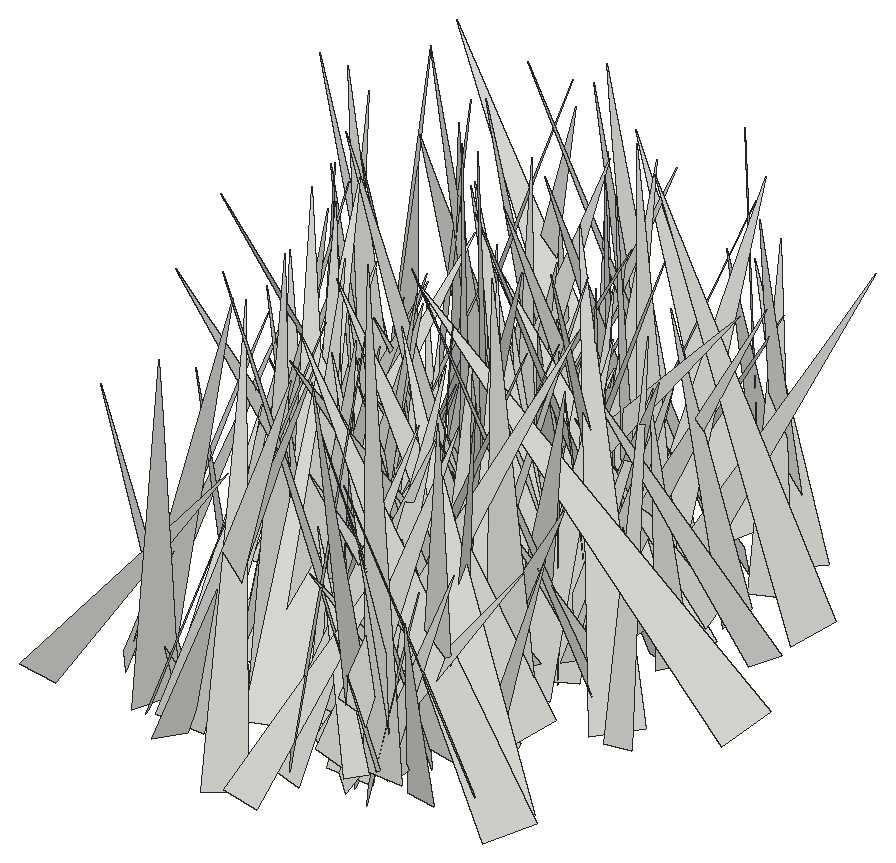
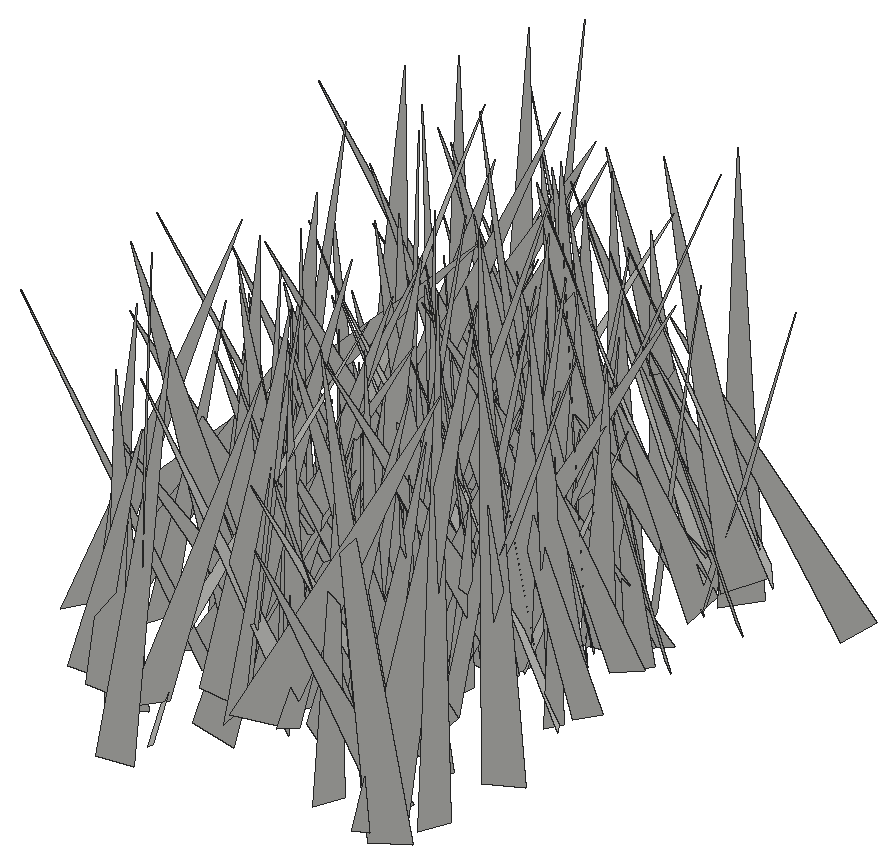
# SketchUp Ruby script. Lengths in inches.
U = 1.inch
M = Sketchup.active_model
def pt(a) = Geom::Point3d.new(a.map { |v| v * U })
def face(e, loops, mat)
  f = e.add_face(loops[0].map { |a| pt(a) })
  loops[1..].each { |l| e.add_face(l.map { |a| pt(a) }).erase! }
  f.material = f.back_material = mat if mat
  f
end
# faces: each face lists its corners as indices into pts; further lists are holes
def faces(e, pts, list, mat = nil) = list.each { |f| face(e, (f[0].is_a?(Array) ? f : [f]).map { |l| l.map { |i| pts[i] } }, mat) }
# xy, xz, yz: faces in a plane at the given z, y or x. An outline is a flat list of corners, or four numbers for a rectangle; further outlines are holes
def ring(l) = l.size == 4 ? [[l[0], l[1]], [l[2], l[1]], [l[2], l[3]], [l[0], l[3]]] : l.each_slice(2).to_a
def flat(e, list, mat, &to3) = list.each { |f| face(e, (f[0].is_a?(Array) ? f : [f]).map { |l| ring(l).map { |u, v| to3.(u, v) } }, mat) }
def xy(e, z, list, mat = nil) = flat(e, list, mat) { |x, y| [x, y, z] }
def xz(e, y, list, mat = nil) = flat(e, list, mat) { |x, z| [x, y, z] }
def yz(e, x, list, mat = nil) = flat(e, list, mat) { |y, z| [x, y, z] }
def lines(e, pts, list) = list.each { |a, b| e.add_line(pt(pts[a]), pt(pts[b])) }
# prism: a flat outline (further loops are holes) pulled along v
def prism(e, loops, v, mat = nil)
  f = face(e, loops, mat); d = Geom::Vector3d.new(v.map { |x| x * U })
  f.pushpull(f.normal.samedirection?(d) ? d.length : -d.length)
end
def box(e, o, s, mat = nil) = prism(e, [[o, [o[0] + s[0], o[1], o[2]], [o[0] + s[0], o[1] + s[1], o[2]], [o[0], o[1] + s[1], o[2]]]], [0, 0, s[2]], mat)
def at(x, y, z, deg = 0) = Geom::Transformation.translation(pt([x, y, z])) * Geom::Transformation.rotation(ORIGIN, Z_AXIS, deg.degrees)
def axes(o, x, y, z) = Geom::Transformation.new([*x, 0, *y, 0, *z, 0, *pt(o).to_a, 1])
def part(name) = M.definitions.add(name)
# library, detail: a bought-in or finely detailed component or shape, given as its bounding box
def library(name, o, s) = part(name).tap { |d| box(d.entities, o, s) }
def detail(e, o, s) = box(e.add_group.entities, o, s)
def put(e, d, t, mat = nil) = e.add_instance(d, t).tap { |i| i.material = mat if mat }
def group(e, t, mat = nil) = e.add_group.tap { |g| g.transformation = t; g.material = mat if mat }.entities
root = M.entities
c1 = part("fur_instance\#9")
p = [[0.8125,0,1.79],[0.67,-0.02,1.48],[0,-0.11,0],[0,0.11,0]]
faces(c1.entities,p,[[0,1,2,3]])
put(root,c1,axes([78.76,74.87,-28.22],[-4.90354,-1.85753,0.89414],[-1.8937,4.97041,-0.05944],[0.81474,0.37312,5.24324]))
put(root,c1,axes([74.27,73.58,-28.22],[3.74419,-3.98525,0.35569],[-3.51637,-3.04515,2.89653],[1.90889,2.20738,4.63803]))
put(root,c1,axes([81.04,83.26,-27.1],[-7.866,-1.33504,0.19154],[-1.32695,7.45779,-2.51268],[-0.24134,2.50839,7.5725]))
put(root,c1,axes([76.8125,81.12,-27.1],[-1.32926,4.80497,0.97182],[4.66035,1.55098,-1.29408],[1.52094,-0.553,4.81456]))
put(root,c1,axes([78.3,80.58,-27.1],[-1.55203,4.86816,1.43833],[5.0761,1.479,0.47157],[-0.03172,-1.51332,5.08777]))
put(root,c1,axes([78.59,81.8,-27.1],[-7.01527,0.64484,2.20419],[0.06996,7.14138,-1.86657],[2.29551,1.75305,6.79307]))
put(root,c1,axes([78.87,84.04,-27.1],[-4.6642,0.46344,0.8289],[0.1067,4.38406,-1.85075],[0.94364,1.79496,4.30631]))
put(root,c1,axes([75.77,77.2,-27.1],[4.35224,4.23695,0.82253],[4.28263,-4.09432,-1.57033],[0.53605,-1.68972,5.86752]))
put(root,c1,axes([76.0625,80.16,-27.1],[4.67492,4.49227,1.13099],[4.6277,-4.45606,-1.42912],[0.20972,-1.8104,6.324]))
put(root,c1,axes([76.66,90.22,-28.22],[7.73874,0.04549,1.82687],[0.5794,-7.60007,-2.26513],[-1.73315,-2.33761,7.39995]))
put(root,c1,axes([77.17,89.34,-27.1],[4.35751,-1.25814,0.68683],[-1.21703,-4.4086,-0.35441],[-0.75729,-0.15444,4.52164]))
put(root,c1,axes([77.69,91.51,-28.22],[6.63906,-4.24471,1.17982],[-3.75911,-6.57064,-2.48644],[-2.29753,-1.51516,7.47745]))
put(root,c1,axes([79.32,82.79,-27.1],[-2.85386,-2.94003,0.13695],[-2.93623,2.85714,0.14971],[0.2028,-0.00613,4.09462]))
put(root,c1,axes([78.6,75.36,-28.22],[-5.00496,1.9066,1.35129],[1.19771,4.83542,-2.3864],[2.00664,1.8693,4.79477]))
put(root,c1,axes([79.34,83.54,-27.1],[-7.46216,1.5868,2.36089],[1.65538,7.81249,-0.01867],[2.31332,-0.47194,7.62898]))
put(root,c1,axes([77.67,83.45,-28.22],[3.91592,-0.46866,0.80636],[-0.26131,-3.89224,-0.99321],[-0.89531,-0.91384,3.81675]))
put(root,c1,axes([77.03,74.16,-27.1],[4.58247,4.01128,0.43645],[4.00699,-4.60163,0.22113],[-0.47421,-0.12046,6.08609]))
put(root,c1,axes([79.05,75.29,-27.1],[-4.90566,2.32822,0.51514],[1.6552,4.17303,-3.098],[1.71648,2.62995,4.45965]))
put(root,c1,axes([77.82,79.22,-28.22],[3.13443,-2.25979,0.73802],[-2.32723,-3.16608,0.18952],[-0.4851,0.5876,3.85946]))
put(root,c1,axes([81.81,83.98,-28.22],[-3.80092,-6.72254,0.0507],[-6.48684,3.65215,-2.05545],[-1.76524,1.05421,7.4441]))
put(root,c1,axes([76,83.94,-27.1],[0.54416,-5.67013,1.84078],[-5.27926,0.40028,2.79359],[2.76917,1.87733,4.9641]))
put(root,c1,axes([78.63,80.76,-27.1],[-4.89725,-3.9807,3.26033],[-4.56553,5.43754,-0.21877],[2.37312,2.24631,6.30723]))
put(root,c1,axes([76.62,87.05,-28.22],[-0.13317,-8.12567,1.45261],[-7.87911,0.55826,2.40046],[2.46092,1.34765,7.76415]))
put(root,c1,axes([77.31,75.09,-27.1],[6.16664,-2.56617,1.31423],[-2.70082,-6.22755,0.51287],[-1.00896,0.98602,6.65955]))
put(root,c1,axes([79.95,81.62,-27.1],[4.59054,6.55576,1.84003],[6.00661,-4.94402,2.62946],[-3.20693,0.124,7.5589]))
put(root,c1,axes([79.47,85.91,-27.1],[-3.91198,-5.41617,1.52932],[-5.50053,4.07361,0.35664],[1.19076,1.02376,6.67167]))
put(root,c1,axes([78.52,80.5625,-27.1],[2.84043,2.51238,0.82611],[2.52394,-2.93724,0.2547],[-0.79009,-0.35083,3.78354]))
put(root,c1,axes([79.33,76.82,-28.22],[-4.6895,-2.45579,1.69505],[-2.43913,4.97359,0.45768],[1.71894,0.35769,5.27378]))
put(root,c1,axes([77.96,74.4,-28.22],[6.0824,-3.06076,1.36011],[-2.97573,-6.23245,-0.71791],[-1.53726,-0.04598,6.77115]))
put(root,c1,axes([78.59,80.53,-27.1],[4.23217,0.79223,1.75299],[1.35483,-4.23497,-1.35698],[-1.36567,-1.74623,4.08626]))
put(root,c1,axes([77.05,91.76,-28.22],[0.9927,-7.18833,2.00129],[-7.23058,-0.4281,2.04891],[1.84279,2.19257,6.96128]))
put(root,c1,axes([78.36,78.8,-28.22],[7.07212,-1.1156,2.41076],[-1.38462,-7.39913,0.63784],[-2.26697,1.03896,7.1311]))
put(root,c1,axes([80.45,81.93,-27.1],[-6.61174,-0.50833,1.66504],[-0.62205,6.79727,-0.39495],[1.62598,0.53342,6.61948]))
put(root,c1,axes([80.125,88.79,-27.1],[-0.83956,4.61048,2.28414],[5.1209,0.52371,0.82514],[-0.50027,-2.37653,4.61309]))
put(root,c1,axes([79.41,74.06,-27.1],[-0.73079,4.32054,0.1844],[4.30671,0.74406,-0.36572],[0.39156,-0.12013,4.36662]))
put(root,c1,axes([79.86,87.125,-28.22],[0.81104,4.54834,1.26147],[4.65262,-0.98593,0.56355],[-0.7949,-1.13006,4.58559]))
put(root,c1,axes([77.7,82.79,-27.1],[3.43659,4.37627,1.35344],[4.55407,-3.08156,-1.59944],[0.49399,-2.03617,5.32951]))
put(root,c1,axes([80.07,85.16,-28.22],[-4.55771,-1.35516,1.4154],[-1.26006,4.77117,0.51063],[1.50069,-0.10962,4.72742]))
put(root,c1,axes([79.25,74.73,-28.22],[5.51307,6.12337,0.96272],[5.81555,-5.55551,2.03274],[-2.14519,0.67601,7.98483]))
put(root,c1,axes([78.45,90.6,-28.22],[1.64053,-3.56149,0.70323],[-3.59089,-1.47867,0.88831],[0.53314,0.99969,3.81922]))
put(root,c1,axes([80.87,81.26,-27.1],[-6.78403,-3.28205,0.63683],[-2.89291,6.48484,2.60352],[1.67585,-2.09175,7.07224]))
put(root,c1,axes([83.32,90.05,-27.1],[-5.71693,5.39586,0.3581],[5.20349,5.34707,2.50186],[-1.47216,-2.05434,7.45247]))
put(root,c1,axes([80.95,83.7,-28.22],[-4.35702,1.54483,0.37411],[1.45493,4.3157,-0.87633],[0.64002,0.7059,4.53896]))
put(root,c1,axes([77.67,83.2,-28.22],[4.98455,3.49636,0.32674],[3.50629,-4.92427,-0.79656],[0.19289,-0.83908,6.03621]))
put(root,c1,axes([79.35,72.3,-27.1],[3.38601,2.0667,0.33408],[1.88033,-3.28152,1.24252],[-0.92044,0.89903,3.76728]))
put(root,c1,axes([80.5,80.37,-28.22],[-3.8802,0.07929,1.10053],[0.11582,4.03064,0.11798],[1.09728,-0.14508,3.87922]))
put(root,c1,axes([79.5,82.96,-27.1],[6.78257,3.66457,1.14232],[2.83952,-6.35069,3.51329],[-2.58286,2.6414,6.86216]))
put(root,c1,axes([77.94,90.25,-28.22],[4.34648,-1.55951,0.20323],[-1.53377,-4.07129,1.56122],[0.34774,1.53551,4.34586]))
put(root,c1,axes([78.38,78.01,-28.22],[-0.73588,7.38124,0.25307],[6.98236,0.77818,-2.39362],[2.40696,-0.00075,7.02103]))
put(root,c1,axes([80.36,83.2,-28.22],[5.2038,5.70361,2.35891],[5.67233,-5.63566,1.11317],[-2.43315,-0.93989,7.64013]))
put(root,c1,axes([79.96,90.97,-28.22],[4.81176,-1.3762,1.70282],[-1.26945,-5.10354,-0.53746],[-1.78382,-0.0803,4.97575]))
put(root,c1,axes([82.38,88.38,-28.22],[-3.32037,-5.8988,2.51801],[-6.36421,2.67847,-2.11746],[-0.7956,3.19234,6.42939]))
put(root,c1,axes([78.86,89.73,-28.22],[2.1882,-4.93746,0.79161],[-4.93819,-1.99768,1.19031],[0.78701,1.19336,5.26781]))
put(root,c1,axes([81.52,86.59,-28.22],[1.26749,-5.25605,0.55346],[-5.00773,-1.37633,-1.60227],[-1.68968,0.13629,5.16385]))
put(root,c1,axes([80.47,76.65,-28.22],[-0.16128,6.84934,2.86842],[7.42417,0.20732,-0.07764],[0.15166,-2.86546,6.8508]))
put(root,c1,axes([78.57,75.2,-27.1],[5.68273,3.19615,0.64935],[3.24559,-5.67036,-0.49352],[-0.32122,-0.74969,6.50117]))
put(root,c1,axes([81.94,85.8125,-27.1],[-7.67624,-2.38765,2.18106],[-2.53698,7.93,-0.24775],[2.0054,0.89261,8.03519]))
put(root,c1,axes([81.24,81.71,-27.1],[-0.33834,3.74046,0.53618],[3.75079,0.26714,0.50319],[-0.45836,-0.57497,3.72187]))
put(root,c1,axes([80.7,85.74,-27.1],[3.27584,-2.78093,0.2499],[-2.38988,-2.99185,-1.96583],[-1.44378,-1.35736,3.82103]))
put(root,c1,axes([82.16,76.27,-28.22],[-5.1988,6.07272,1.14347],[6.1224,5.26442,-0.12263],[0.83765,-0.78798,7.99315]))
put(root,c1,axes([79.35,82.78,-27.1],[3.86855,-0.79855,0.19754],[-0.81455,-3.85123,0.38332],[-0.11496,0.41562,3.93147]))
put(root,c1,axes([81.46,82.02,-28.22],[-0.43977,4.5707,0.64422],[4.59918,0.3789,0.45132],[-0.39225,-0.6818,4.56957]))
put(root,c1,axes([79.14,88.125,-27.1],[2.35297,-5.60644,2.50548],[-6.03434,-1.6135,2.05656],[1.13856,3.03489,5.72182]))
put(root,c1,axes([82.9,76,-27.1],[-6.0397,-1.24718,1.08354],[-1.47294,5.92489,-1.39057],[0.74831,1.59618,6.00831]))
put(root,c1,axes([79.6875,79.56,-27.1],[5.0608,-1.8582,0.79428],[-1.91101,-5.09708,0.2516],[-0.65714,0.51221,5.38529]))
put(root,c1,axes([79.54,73.09,-28.22],[6.41211,-0.61612,1.30158],[-0.93497,-6.2989,1.62436],[-1.09524,1.77006,6.23347]))
put(root,c1,axes([82.84,71.48,-28.22],[-6.61706,2.95045,0.41304],[2.75432,6.44194,-1.89112],[1.13554,1.56763,6.99387]))
put(root,c1,axes([79.96,87.74,-27.1],[4.40688,2.08061,0.00975],[2.02682,-4.29803,1.08102],[-0.47012,0.97349,4.75194]))
put(root,c1,axes([79.34,73.8125,-28.22],[2.98572,-5.88102,1.99527],[-6.13329,-2.44486,1.97166],[0.97482,2.63026,6.29392]))
put(root,c1,axes([83.88,82.41,-27.1],[-7.9003,-1.05971,0.99848],[-1.05239,7.96314,0.1246],[1.0062,0.00826,7.97008]))
put(root,c1,axes([79.52,80.73,-28.22],[4.01839,-5.64573,1.18023],[-5.73753,-3.76564,1.52164],[0.58986,1.83314,6.76065]))
put(root,c1,axes([82.41,85.7,-28.22],[1.55743,6.34801,1.89562],[6.44853,-1.89902,1.06134],[-1.51893,-1.55328,6.44953]))
put(root,c1,axes([82.76,73.87,-27.1],[-4.41357,6.91206,0.00056],[6.86097,4.38103,-0.99489],[0.83882,0.53496,8.14041]))
put(root,c1,axes([82.54,76.4,-28.22],[-1.87564,7.62096,1.95831],[7.8685,1.80971,0.49369],[-0.027,-2.0194,7.83284]))
put(root,c1,axes([82.36,89.85,-27.1],[-3.76395,0.54517,1.33918],[0.93594,3.7652,1.09781],[1.1021,-1.33566,3.64133]))
put(root,c1,axes([79.06,89.62,-28.22],[5.13352,5.29295,1.04527],[5.31008,-4.70157,-2.27141],[0.95446,-2.31104,7.01492]))
put(root,c1,axes([83.82,77.97,-28.22],[-1.56415,5.71782,0.81541],[5.62888,1.31989,1.54221],[-1.29382,-1.17019,5.72377]))
put(root,c1,axes([80.8125,79.18,-27.1],[3.7872,-0.0255,0.26622],[0.02172,-3.73751,-0.66706],[-0.26655,-0.66693,3.72808]))
put(root,c1,axes([82.58,75.08,-27.1],[-5.70861,3.53079,2.01517],[3.32922,6.05385,-1.17592],[2.33318,0.00055,6.60847]))
put(root,c1,axes([82.73,80.1875,-27.1],[0.53786,-3.60504,0.14249],[-3.55289,-0.5543,-0.6129],[-0.62738,0.04841,3.59304]))
put(root,c1,axes([80.73,89.14,-27.1],[5.43533,-0.93824,0.08866],[-0.80913,-4.91198,-2.3767],[-0.48317,-2.32876,4.97739]))
put(root,c1,axes([81.07,77.69,-28.22],[2.15737,-6.51602,1.69287],[-6.69271,-1.88316,1.28061],[0.7294,1.99342,6.74336]))
put(root,c1,axes([86.87,73.8125,-27.1],[-6.97142,-3.26118,0.0354],[-2.96258,6.29742,-3.28677],[-1.3637,2.99072,6.9594]))
put(root,c1,axes([81.07,85.01,-28.22],[5.44463,0.12063,0.24069],[0.04962,-5.23956,1.50366],[-0.26462,1.49964,5.23426]))
put(root,c1,axes([80.71,84.64,-27.1],[6.6655,-1.52718,0.22941],[-1.49066,-6.62814,-0.81212],[-0.40351,-0.74118,6.78982]))
put(root,c1,axes([84.09,90.09,-27.1],[-6.8866,-1.44069,2.04712],[-1.4724,7.17733,0.09795],[2.02444,0.3193,7.035]))
put(root,c1,axes([84.39,80.79,-28.22],[-7.45834,-2.27512,2.73301],[-2.96816,7.48025,-1.87304],[1.95846,2.67246,7.56933]))
put(root,c1,axes([83.48,85.23,-27.1],[-3.08367,2.72536,1.78242],[3.08151,3.23588,0.38343],[1.05304,-1.48834,4.09751]))
put(root,c1,axes([84.33,87.04,-28.22],[-6.55431,0.09701,1.7896],[-0.34688,6.588,-1.62754],[1.75834,1.66126,6.34976]))
put(root,c1,axes([83.85,84.11,-28.22],[0.37183,-3.94608,0.38846],[-3.8933,-0.43727,-0.71534],[-0.75144,0.31297,3.89847]))
put(root,c1,axes([84.875,89.6875,-27.1],[-1.73257,6.85044,2.42635],[7.20837,1.30251,1.46979],[-0.92468,-2.68187,6.91158]))
put(root,c1,axes([82.66,84.1,-28.22],[-0.63847,4.33122,0.11328],[4.14955,0.64421,-1.24344],[1.2464,0.07394,4.19773]))
put(root,c1,axes([83.06,80.74,-27.1],[4.36466,2.86173,1.95624],[3.18404,-4.55325,-0.44325],[-1.3705,-1.46462,5.20032]))
put(root,c1,axes([85.26,83.08,-27.1],[-5.2406,4.407,1.34408],[4.57378,5.22157,0.71269],[0.55566,-1.41624,6.81011]))
put(root,c1,axes([87.54,89.21,-27.1],[-7.14593,-4.06809,0.00282],[-3.91681,6.87864,-2.22635],[-1.09909,1.93614,7.91562]))
put(root,c1,axes([84.1,84.14,-28.22],[-3.37943,-0.96857,0.84627],[-0.6019,3.29348,1.36586],[1.13667,-1.13567,3.23931]))
put(root,c1,axes([84.03,87.23,-27.1],[-0.63245,-3.70623,0.66325],[-3.76509,0.62047,-0.12308],[-0.01169,0.67448,3.75779]))
put(root,c1,axes([85.34,88.22,-28.22],[-0.04463,-6.97717,1.39975],[-6.92736,-0.27772,-1.60522],[-1.62845,1.37265,6.79015]))
put(root,c1,axes([83.9,88.21,-28.22],[3.78368,4.97369,3.03573],[5.56614,-4.15585,-0.12867],[-1.72376,-2.50217,6.24798]))
put(root,c1,axes([84.41,86.54,-28.22],[-2.40754,3.72637,1.88833],[4.14407,2.40561,0.53634],[0.52762,-1.89079,4.40391]))
put(root,c1,axes([82.66,77.62,-27.1],[-2.78435,-5.66723,3.39056],[-5.97834,3.72634,1.319],[2.80584,2.3158,6.17497]))
put(root,c1,axes([81.21,81.07,-28.22],[7.73901,0.54751,0.09462],[0.50511,-7.48314,1.98706],[-0.23147,1.9758,7.49957]))
put(root,c1,axes([85.05,89.98,-28.22],[-0.92127,-7.60318,0.93237],[-7.64439,0.85236,-0.60268],[-0.49091,0.99576,7.63504]))
put(root,c1,axes([83.86,76.51,-28.22],[-3.43259,1.11019,2.13702],[1.24058,4.00441,-0.08763],[2.06406,-0.56053,3.60659]))
put(root,c1,axes([86.41,91.24,-27.1],[-6.01632,2.22797,0.81671],[2.32649,5.97644,0.83455],[0.46722,-1.07014,6.36109]))
put(root,c1,axes([86.2,80.86,-27.1],[2.18391,-6.70079,0.42323],[-6.08063,-2.16263,-2.86325],[-2.84706,-0.52116,6.43986]))
put(root,c1,axes([86.59,88.07,-28.22],[-2.69174,-3.80387,0.07847],[-3.66679,2.56798,-1.29661],[-1.01502,0.8106,4.47591]))
put(root,c1,axes([82.83,88.76,-27.1],[5.42276,2.60915,0.23648],[2.58182,-5.41452,0.53583],[-0.44475,0.3811,5.9939]))
put(root,c1,axes([85.51,80.41,-27.1],[-6.98093,-2.98191,2.95578],[-3.56155,7.24267,-1.10492],[2.22346,2.23913,7.51028]))
put(root,c1,axes([86.6,75.18,-27.1],[-5.80582,1.67481,0.45332],[1.66732,5.82342,-0.1609],[0.48013,0.02943,6.04042]))
put(root,c1,axes([85.71,84.58,-27.1],[-3.47043,-1.20582,0.35373],[-1.16309,3.47557,0.43669],[0.47575,-0.29913,3.64791]))
put(root,c1,axes([84.6,77.88,-27.1],[2.87799,2.64757,1.74089],[2.94858,-3.09885,-0.16173],[-1.16026,-1.30792,3.90721]))
put(root,c1,axes([83.55,73.28,-28.22],[0.68062,5.93772,0.86921],[5.89172,-0.495,-1.23203],[1.14003,-0.98679,5.84823]))
put(root,c1,axes([83.43,78.71,-28.22],[5.03516,3.5658,0.22039],[3.50469,-5.00395,0.89105],[-0.69327,0.6016,6.10523]))
put(root,c1,axes([85.06,83.76,-27.1],[-1.60634,4.05647,0.77587],[4.09581,1.67158,-0.25963],[0.53033,-0.623,4.35521]))
put(root,c1,axes([83.49,71.4,-28.22],[-2.11402,4.56513,0.60738],[3.84978,2.11854,-2.52378],[2.52756,0.59144,4.35202]))
put(root,c1,axes([84.43,72.55,-27.1],[5.20843,4.28763,1.83578],[4.29945,-5.48037,0.60158],[-1.80791,-0.68076,6.71935]))
put(root,c1,axes([86.52,73,-27.1],[-0.98772,3.5916,0.11089],[3.35733,0.88143,1.35606],[-1.28071,-0.45933,3.46934]))
put(root,c1,axes([88.375,86.31,-28.22],[-6.39943,2.86094,0.01202],[2.71801,6.07041,2.2137],[-0.89308,-2.0256,6.65111]))
put(root,c1,axes([85.47,78.5,-27.1],[-4.49774,2.41965,1.22715],[2.26445,4.65664,-0.88215],[1.49428,0.22634,5.03052]))
put(root,c1,axes([82.98,75.65,-27.1],[2.29321,-4.71361,1.70331],[-4.8602,-1.63403,2.02152],[1.22385,2.34308,4.83635]))
put(root,c1,axes([84.94,86.23,-27.1],[-5.03968,3.97301,2.20808],[3.85689,5.48236,-1.06156],[2.40517,-0.46656,6.329]))
put(root,c1,axes([87.78,85.45,-28.22],[-4.08084,-6.31933,0.93728],[-6.28934,3.77891,-1.90517],[-1.12095,1.80323,7.27719]))
put(root,c1,axes([85.7,84.49,-27.1],[-3.90689,0.46662,1.17538],[0.26281,4.03296,-0.72751],[1.23701,0.61693,3.86682]))
put(root,c1,axes([85.11,86.32,-28.22],[1.4103,3.34023,0.25009],[3.32818,-1.428,0.30438],[-0.37801,-0.11091,3.61295]))
put(root,c1,axes([86.65,77.71,-27.1],[-4.86866,0.51762,1.11395],[0.97098,4.41082,2.19421],[0.75234,-2.34296,4.3769]))
put(root,c1,axes([86.41,82.62,-28.22],[-5.37291,2.30629,0.61766],[1.96946,5.14098,-2.06404],[1.34972,1.6793,5.47055]))
put(root,c1,axes([87.89,77.5,-28.22],[-5.88175,-1.50758,0.15009],[-1.51502,5.85044,-0.60606],[-0.00586,0.62434,6.04156]))
put(root,c1,axes([86.38,77.99,-28.22],[-4.21387,-1.59887,0.24339],[-1.27519,3.70248,2.24451],[0.99474,-2.02671,3.90836]))
put(root,c1,axes([85.84,84.82,-28.22],[-3.08736,-2.6391,1.38175],[-2.74426,3.29386,0.15946],[1.15895,0.7691,4.05847]))
put(root,c1,axes([83.46,77.81,-27.1],[6.47298,0.85818,0.33872],[0.84258,-6.4766,0.30739],[-0.37587,0.26066,6.52238]))
put(root,c1,axes([85.18,75.14,-28.22],[-6.68782,-2.79113,3.18251],[-2.04813,7.34131,2.13449],[3.70459,-0.98003,6.92541]))
put(root,c1,axes([86.66,78.6875,-28.22],[-3.82919,5.78151,1.38736],[5.88668,3.91838,-0.08139],[0.83523,-1.11076,6.93412]))
put(root,c1,axes([85.125,74.44,-28.22],[-1.23701,6.48468,1.94316],[6.59867,1.59608,-1.12573],[1.51147,-1.6609,6.50492]))
put(root,c1,axes([87.62,75.09,-27.1],[-4.41159,-3.54695,0.73212],[-3.61607,4.3782,-0.57829],[0.20221,0.91078,5.63104]))
put(root,c1,axes([88.93,78.1,-27.1],[-7.28796,2.50197,0.93453],[2.66483,6.99355,2.0583],[0.17855,-2.25345,7.42547]))
put(root,c1,axes([86.64,80.25,-28.22],[-3.91308,1.33626,1.31278],[1.41439,4.10109,0.04154],[1.2282,-0.46546,4.13474]))
put(root,c1,axes([85.39,78.97,-27.1],[4.30738,5.01035,0.65824],[4.94004,-4.35705,0.83813],[-1.06435,0.05398,6.55397]))
put(root,c1,axes([81.13,85.63,-27.1],[5.03462,6.0848,0.40692],[5.07887,-3.8915,-4.64748],[3.37572,-3.22012,6.38538]))
put(root,c1,axes([87.15,73.44,-27.1],[1.25442,7.48082,2.76942],[7.81491,-1.71475,1.09211],[-1.59984,-2.51056,7.50623]))
put(root,c1,axes([86.32,85.08,-28.22],[2.40837,2.51325,1.53163],[2.71206,-2.66382,0.10655],[-1.14326,-1.0248,3.47927]))
put(root,c1,axes([84.38,86.2,-28.22],[5.53562,0.75174,0.06867],[0.66774,-5.11345,2.14935],[-0.35205,2.12143,5.1564]))
put(root,c1,axes([87.33,86.05,-27.1],[-0.74799,6.94474,2.29097],[7.27165,0.46217,0.97314],[-0.77532,-2.36525,6.91678]))
put(root,c1,axes([87.65,84.49,-27.1],[-6.31895,-1.30533,1.91515],[-1.71826,6.37081,-1.32708],[1.5554,1.73484,6.31441]))
put(root,c1,axes([86.04,82.98,-28.22],[-3.42009,-2.62307,1.97794],[-2.56254,3.91671,0.76324],[2.05575,0.51835,4.24205]))
put(root,c1,axes([86.09,91.59,-28.22],[-2.58943,-3.13022,0.07236],[-2.65217,2.2427,2.10831],[1.66419,-1.2964,3.47253]))
put(root,c1,axes([88.25,81.65,-27.1],[-5.65228,-5.31186,0.60473],[-5.29476,5.68375,0.43618],[0.73959,0.09466,7.74428]))
put(root,c1,axes([85.48,80.67,-28.22],[6.82922,2.21825,1.16198],[1.82522,-6.72015,2.10172],[-1.71447,1.68168,6.86597]))
put(root,c1,axes([86.32,92.9375,-28.22],[0.33482,-6.22736,0.74708],[-6.26175,-0.28913,0.39628],[0.3585,0.76592,6.22375]))
put(root,c1,axes([83.875,86.93,-28.22],[1.01842,-6.5564,0.3467],[-5.92672,-0.76709,2.90332],[2.82498,0.75429,5.9661]))
put(root,c1,axes([86.15,81.41,-28.22],[-2.07384,5.25709,1.74566],[5.26815,2.4479,-1.11335],[1.712,-1.16445,5.54061]))
put(root,c1,axes([88.0625,78.33,-28.22],[-4.14982,-0.72477,0.23143],[-0.53834,3.70403,1.94686],[0.53763,-1.88541,3.73578]))
put(root,c1,axes([90.83,74.72,-28.22],[-4.49913,6.58347,1.21187],[6.27218,3.63575,3.53468],[-2.33889,-2.91414,7.14775]))
put(root,c1,axes([86.67,91.48,-27.1],[-4.90081,-4.60842,2.76686],[-4.75517,5.4628,0.67611],[2.50627,1.35324,6.69315]))
put(root,c1,axes([85.42,73.32,-27.1],[0.44188,5.84269,1.52194],[5.83939,-0.02571,-1.59672],[1.53457,-1.58458,5.63763]))
put(root,c1,axes([85.09,82.86,-27.1],[0.27487,-5.90315,0.86813],[-5.62576,0.03312,2.00651],[1.98787,0.91,5.55848]))
put(root,c1,axes([87.48,74.09,-27.1],[-3.67755,-0.2078,1.11626],[-0.0694,3.8179,0.48208],[1.13331,-0.4405,3.65173]))
put(root,c1,axes([86.86,83.64,-27.1],[5.38301,1.51294,2.42188],[1.75431,-5.82988,-0.25732],[-2.2532,-0.92457,5.58566]))
put(root,c1,axes([86.12,83.38,-27.1],[1.17442,4.10835,0.87727],[4.16659,-1.02282,-0.78793],[0.5364,-1.0501,4.19964]))
put(root,c1,axes([86.23,85.77,-27.1],[-2.59583,-7.17613,0.91864],[-6.91744,2.74775,1.9178],[2.11891,0.17907,7.38629]))
put(root,c1,axes([84.99,80.95,-27.1],[1.43751,-4.12245,0.23292],[-3.7226,-1.18725,1.96162],[1.78636,0.84328,3.90039]))
put(root,c1,axes([84.02,74.96,-28.22],[2.96543,7.80813,0.73471],[7.53088,-2.61577,-2.59693],[2.18919,-1.57838,7.9383]))
put(root,c1,axes([86.35,83.17,-28.22],[4.97283,-0.90694,1.68915],[-1.45035,-4.85051,1.66547],[-1.25389,2.01364,4.77261]))
put(root,c1,axes([87.36,82.8125,-27.1],[-3.37323,-1.69913,0.74168],[-1.13548,3.11072,1.96213],[1.46554,-1.50074,3.22735]))
put(root,c1,axes([88.72,86.8,-27.1],[-4.09373,-0.36711,0.23804],[-0.24891,3.79616,1.57392],[0.35983,-1.55061,3.79686]))
put(root,c1,axes([86.18,73.95,-28.22],[3.53808,2.09554,0.91862],[2.27584,-3.39762,-1.01485],[-0.23603,-1.34836,3.98489]))
put(root,c1,axes([90.34,75.1875,-28.22],[-6.09178,4.42452,0.24879],[4.41982,6.03543,0.88707],[-0.32169,-0.86331,7.47659]))
put(root,c1,axes([86.57,86.375,-27.1],[-2.09917,6.50868,2.06271],[6.47308,2.58358,-1.56477],[2.17184,-1.40938,6.65739]))
put(root,c1,axes([85.5,83.83,-28.22],[5.89458,-2.32049,1.52507],[-2.76984,-5.16651,2.8446],[-0.1962,3.22166,5.6603]))
put(root,c1,axes([86.32,77.83,-27.1],[6.10646,0.88523,1.50787],[1.27518,-6.00248,-1.64024],[-1.19633,-1.87958,5.94829]))
put(root,c1,axes([89.03,90.9375,-27.1],[-2.03282,4.17049,1.29504],[4.34211,1.77825,1.08919],[-0.46493,-1.62705,4.50988]))
put(root,c1,axes([89.64,74.48,-27.1],[-3.75562,-3.58045,0.3486],[-3.58145,3.67402,-0.84892],[-0.33818,0.85312,5.11895]))
put(root,c1,axes([87.93,78.46,-27.1],[1.68119,-6.78383,2.85706],[-7.30642,-1.89388,-0.19753],[-0.89411,2.72073,6.98625]))
put(root,c1,axes([87.94,90.34,-28.22],[-2.39493,4.93051,2.15105],[5.27679,2.61079,-0.10925],[1.04521,-1.88321,5.4803]))
put(root,c1,axes([84.94,74.24,-28.22],[3.04424,4.32162,0.01521],[3.85535,-2.70735,-2.39804],[1.95268,-1.39208,4.71097]))
put(root,c1,axes([89.53,81.3125,-28.22],[-6.04844,4.67756,1.28768],[4.75602,6.12308,0.0974],[0.95811,-0.86582,7.6455]))
put(root,c1,axes([87.9375,91.49,-27.1],[-0.39451,-5.89979,1.57703],[-6.09619,0.47415,0.24879],[0.36204,1.55494,5.90773]))
put(root,c1,axes([93.56,82.25,-27.1],[-5.86481,5.71927,0.12396],[4.62698,4.63811,4.91939],[-3.36399,-3.59156,6.55024]))
put(root,c1,axes([86.79,73.69,-27.1],[-0.2038,-3.57727,1.86557],[-3.68837,0.92217,1.36537],[1.63497,1.63446,3.31273]))
put(root,c1,axes([87.42,75.58,-27.1],[0.11264,-6.37998,1.60761],[-6.5012,0.13924,1.0081],[1.01142,1.60553,6.30084]))
put(root,c1,axes([87.57,74.67,-28.22],[0.30074,-4.21199,0.28121],[-4.14735,-0.24225,0.80695],[0.78703,0.33293,4.14489]))
put(root,c1,axes([88.37,85.37,-28.22],[3.6689,-2.8215,1.45683],[-2.81207,-3.92099,-0.512],[-1.47496,0.45716,4.59995]))
put(root,c1,axes([89.28,87.16,-27.1],[-5.12264,0.34016,1.65759],[0.60899,5.30124,0.79415],[1.57874,-0.94118,5.07212]))
put(root,c1,axes([87.99,76.89,-28.22],[3.72364,-1.08643,0.80362],[-1.21362,-3.72465,0.58799],[-0.59435,0.79892,3.83407]))
put(root,c1,axes([90.08,80.64,-28.22],[1.19098,5.93826,0.851],[5.76454,-1.37303,1.51343],[-1.66049,-0.50738,5.86438]))
put(root,c1,axes([91.57,87.84,-27.1],[-7.37091,1.53228,0.84327],[1.65266,7.29739,1.18581],[0.57246,-1.33774,7.43452]))
put(root,c1,axes([86.18,88.69,-27.1],[3.46284,5.45761,0.55951],[5.19477,-3.049,-2.40992],[1.76435,-1.73432,5.99742]))
put(root,c1,axes([91.48,85.73,-27.1],[0.83306,-5.07313,1.39633],[-4.3947,-1.44829,-2.63999],[-2.89363,0.73905,4.41148]))
